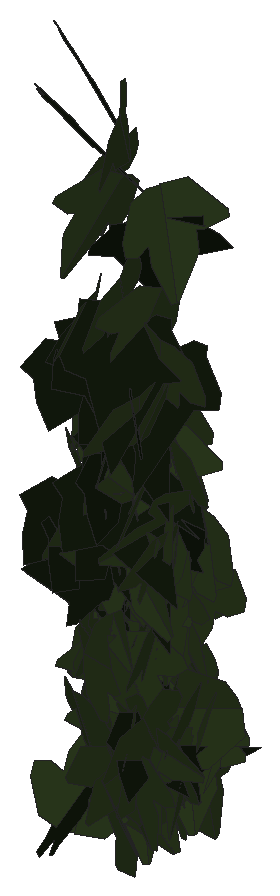
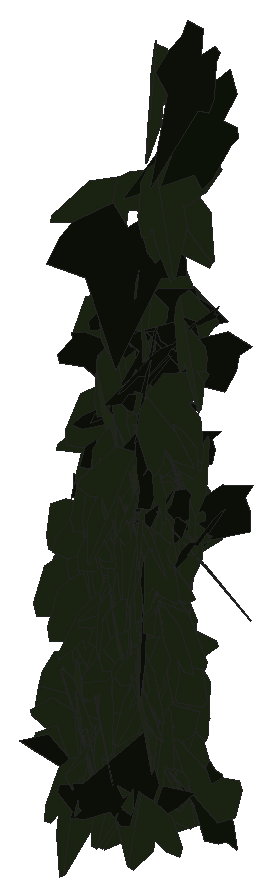
# SketchUp Ruby script. Lengths in inches.
U = 1.inch
M = Sketchup.active_model
def pt(a) = Geom::Point3d.new(a.map { |v| v * U })
def face(e, loops, mat)
  f = e.add_face(loops[0].map { |a| pt(a) })
  loops[1..].each { |l| e.add_face(l.map { |a| pt(a) }).erase! }
  f.material = f.back_material = mat if mat
  f
end
# faces: each face lists its corners as indices into pts; further lists are holes
def faces(e, pts, list, mat = nil) = list.each { |f| face(e, (f[0].is_a?(Array) ? f : [f]).map { |l| l.map { |i| pts[i] } }, mat) }
# xy, xz, yz: faces in a plane at the given z, y or x. An outline is a flat list of corners, or four numbers for a rectangle; further outlines are holes
def ring(l) = l.size == 4 ? [[l[0], l[1]], [l[2], l[1]], [l[2], l[3]], [l[0], l[3]]] : l.each_slice(2).to_a
def flat(e, list, mat, &to3) = list.each { |f| face(e, (f[0].is_a?(Array) ? f : [f]).map { |l| ring(l).map { |u, v| to3.(u, v) } }, mat) }
def xy(e, z, list, mat = nil) = flat(e, list, mat) { |x, y| [x, y, z] }
def xz(e, y, list, mat = nil) = flat(e, list, mat) { |x, z| [x, y, z] }
def yz(e, x, list, mat = nil) = flat(e, list, mat) { |y, z| [x, y, z] }
def lines(e, pts, list) = list.each { |a, b| e.add_line(pt(pts[a]), pt(pts[b])) }
# prism: a flat outline (further loops are holes) pulled along v
def prism(e, loops, v, mat = nil)
  f = face(e, loops, mat); d = Geom::Vector3d.new(v.map { |x| x * U })
  f.pushpull(f.normal.samedirection?(d) ? d.length : -d.length)
end
def box(e, o, s, mat = nil) = prism(e, [[o, [o[0] + s[0], o[1], o[2]], [o[0] + s[0], o[1] + s[1], o[2]], [o[0], o[1] + s[1], o[2]]]], [0, 0, s[2]], mat)
def at(x, y, z, deg = 0) = Geom::Transformation.translation(pt([x, y, z])) * Geom::Transformation.rotation(ORIGIN, Z_AXIS, deg.degrees)
def axes(o, x, y, z) = Geom::Transformation.new([*x, 0, *y, 0, *z, 0, *pt(o).to_a, 1])
def part(name) = M.definitions.add(name)
# library, detail: a bought-in or finely detailed component or shape, given as its bounding box
def library(name, o, s) = part(name).tap { |d| box(d.entities, o, s) }
def detail(e, o, s) = box(e.add_group.entities, o, s)
def put(e, d, t, mat = nil) = e.add_instance(d, t).tap { |i| i.material = mat if mat }
def group(e, t, mat = nil) = e.add_group.tap { |g| g.transformation = t; g.material = mat if mat }.entities
root = M.entities
M.materials.add("efeu1").color = [18, 25, 13]
M.materials.add("efeu2").color = [43, 57, 29]
c1 = part("ivyleaf_10")
p = [[0,0.5,-0.03],[-0.0625,2.02,-0.43],[-0.19,2.01,-0.46],[-0.54,1.05,-0.29],[-0.52,0.625,-0.18],[-0.83,0.76,-0.28],
  [-1.16,0.64,-0.33],[-1.15,0.33,-0.24],[-0.77,-0.39,0.02],[-0.3,-0.51,0.16],[0.04,-0.48,0.23],[-0.02,2.01,-0.4375],
  [-0.06,2.01,-0.43],[0.04,-0.49,0.23],[0.67,-0.49,0.14],[1.38,0.36,-0.2],[1.375,0.51,-0.24],[0.81,0.65,-0.19],
  [0.62,0.59,-0.15],[0.6,1.09,-0.28],[0.5,1.23,-0.31]]
faces(c1.entities,p,[[0,1,2,3,4,5,6,7,8,9,10],[11,12,0,13,14,15,16,17,18,19,20]],"efeu2")
c2 = part("ivyleaf_9")
p = [[1.54,2.16,1.25],[1.36,2.04,1.19],[-0.21,0.99,0.68],[-0.71,1.11,0.82],[-0.85,0.86,0.67],[-0.8,0.17,0.21],
  [-0.9,-0.01,0.1],[-0.67,-0.16,-0.02],[-0.08,-0.08,-0.05],[-0.03,-0.6,-0.4],[0.65,-0.88,-0.66],[0.83,-0.6,-0.49],
  [1.29,-0.42,-0.43],[1.8125,-0.07,-0.26],[1.21,0.44,0.15]]
faces(c2.entities,p,[[0,1,2,3,4,5,6,7,8,9,10,11,12,13,14]],"efeu1")
put(root,c1,axes([21.54,225.2,216.51],[0.41604,-0.27169,0.05558],[0.08058,0.02255,-0.49295],[0.26536,0.41913,0.06255]))
put(root,c1,axes([21.65,225.15,219.01],[0.01266,-0.40962,0.28645],[0.04495,-0.28445,-0.40874],[0.49781,0.0361,0.02962]))
put(root,c1,axes([21.73,225.11,215.11],[-0.42278,0.2511,0.09058],[-0.10121,0.00622,-0.48961],[-0.24701,-0.43233,0.04557]))
put(root,c1,axes([21.71,225.37,215.82],[0.1972,-0.44181,-0.12615],[-0.03153,0.12394,-0.48337],[0.45839,0.1986,0.02102]))
put(root,c1,axes([21.59,225.14,215.95],[-0.16549,-0.37731,-0.28328],[0.18997,0.22151,-0.40601],[0.43188,-0.24201,0.07005]))
put(root,c1,axes([21.7,224.63,219.89],[0.14778,-0.47571,-0.04311],[0.00221,0.0458,-0.49789],[0.47766,0.14696,0.01564]))
put(root,c1,axes([21.59,224.64,213.92],[0.38502,0.29053,-0.13174],[0.10689,0.07705,0.48233],[0.30056,-0.39957,-0.00277]))
put(root,c2,axes([21.44,224.42,222.3125],[0.47565,-0.15225,-0.02409],[-0.00548,0.06139,-0.49619],[0.15404,0.47228,0.05674]))
put(root,c1,axes([21.7,225.26,216.42],[-0.39747,-0.26793,-0.14223],[0.10687,0.09572,-0.47898],[0.28389,-0.41116,-0.01882]))
put(root,c1,axes([21.74,224.64,217.54],[-0.04796,-0.48317,-0.11937],[0.03109,0.11678,-0.48518],[0.49672,-0.05396,0.01884]))
put(root,c2,axes([21.59,224.6,217.65],[-0.01697,-0.37042,-0.33541],[-0.00806,0.33576,-0.3704],[0.49965,-0.00717,-0.01737]))
put(root,c2,axes([21.69,224.17,213.86],[-0.20042,0.45805,-0.0044],[-0.00475,0.00272,0.49997],[0.45805,0.20045,0.00326]))
put(root,c1,axes([22.02,224.84,217.42],[0.04947,0.04496,-0.49551],[-0.32133,0.38307,0.00268],[0.37987,0.31818,0.06679]))
put(root,c2,axes([21.71,224.43,222.99],[0.40824,-0.03682,-0.28633],[-0.28129,0.06078,-0.40888],[0.06492,0.49492,0.02891]))
put(root,c1,axes([21.82,225.16,214.95],[-0.14194,-0.42822,0.21559],[-0.00134,-0.22449,-0.44677],[0.47943,-0.12741,0.06258]))
put(root,c2,axes([21.57,224.68,217.2],[0.22108,-0.41378,-0.17295],[-0.08343,0.15151,-0.46913],[0.44064,0.23629,-0.00205]))
put(root,c1,axes([21.81,224.63,216.55],[0.04249,0.01142,-0.49806],[-0.00091,0.49987,0.01138],[0.49819,-0.00006,0.0425]))
put(root,c2,axes([21.97,224.96,216.85],[0.06294,-0.03259,-0.49495],[-0.45396,0.19727,-0.07072],[0.19989,0.45828,-0.00476]))
put(root,c1,axes([21.75,224.89,215.46],[-0.19102,0.45911,0.0522],[-0.01529,0.05018,-0.49724],[-0.46182,-0.19156,-0.00513]))
put(root,c1,axes([21.78,225.29,217.32],[-0.49192,0.07312,-0.05167],[0.04949,-0.01842,-0.4972],[-0.07462,-0.49428,0.01088]))
put(root,c1,axes([21.84,224.9,221.59],[0.02564,-0.49813,-0.03474],[-0.00713,0.03442,-0.49876],[0.49929,0.02607,-0.00533]))
put(root,c1,axes([21.71,225.31,215.92],[0.35958,-0.34514,0.03978],[0.09029,0.03755,-0.49035],[0.33549,0.35982,0.08933]))
put(root,c1,axes([21.81,224.4375,215.25],[-0.44392,0.23002,-0.00536],[0.00529,-0.00145,-0.49997],[-0.23002,-0.44395,-0.00115]))
put(root,c2,axes([22.15,224.38,217.12],[-0.34255,0.29401,0.21497],[-0.17815,0.12215,-0.45093],[-0.31768,-0.38553,0.02107]))
put(root,c1,axes([21.74,225.46,215.76],[0.38872,-0.28553,0.13181],[0.10715,-0.07677,-0.48231],[0.29567,0.40321,0.00151]))
put(root,c1,axes([21.55,224.7,217.75],[-0.13534,-0.00274,0.48133],[0.44109,-0.20086,0.12288],[0.19268,0.45787,0.05679]))
put(root,c1,axes([21.92,224.92,215.84],[-0.17482,-0.44912,0.13316],[0.01365,-0.14695,-0.47772],[0.46824,-0.1634,0.06364]))
put(root,c1,axes([21.88,225.1875,216.64],[0.14766,-0.46817,-0.09494],[0.01371,0.10348,-0.48898],[0.4775,0.1418,0.0434]))
put(root,c1,axes([21.93,224.7,221.32],[-0.03902,-0.42987,0.25238],[-0.0208,-0.25152,-0.43163],[0.49804,-0.04418,0.00175]))
put(root,c2,axes([22.04,225.5,214.16],[-0.41951,-0.23548,0.13624],[0.13386,0.03932,0.48014],[-0.23684,0.43932,0.03005]))
put(root,c1,axes([21.84,225.3,216.17],[0.12222,0.48453,-0.01723],[-0.05019,-0.00503,-0.49745],[-0.48223,0.12332,0.04741]))
put(root,c1,axes([22.16,224.96,218.28],[-0.42118,0.09296,0.25292],[-0.26479,-0.05576,-0.42045],[-0.04996,-0.48811,0.0962]))
put(root,c1,axes([21.82,224.63,215.86],[-0.24361,0.28524,0.33059],[0.22257,-0.24457,0.37503],[0.37566,0.32988,-0.00782]))
put(root,c1,axes([21.99,224.77,217.17],[-0.19886,-0.45215,0.07755],[0.00778,-0.08783,-0.49216],[0.45869,-0.19454,0.04196]))
put(root,c1,axes([21.92,225.14,217.04],[0.14819,-0.44913,-0.16223],[0.05568,0.18496,-0.46118],[0.47428,0.11862,0.10483]))
put(root,c1,axes([22,224.88,216.875],[0.446,-0.17424,-0.14396],[-0.13368,0.05342,-0.47883],[0.18224,0.4656,0.00107]))
put(root,c1,axes([21.98,224.76,216.26],[-0.02511,-0.43788,-0.24007],[0.01663,0.23951,-0.43859],[0.49909,-0.03002,0.00253]))
put(root,c1,axes([21.91,225.125,217.48],[0.3805,-0.32173,0.04135],[0.04906,-0.00593,-0.49755],[0.32065,0.38269,0.02706]))
put(root,c1,axes([22.02,225.25,216.35],[-0.02831,-0.49885,-0.01868],[0.0001,0.0187,-0.49965],[0.4992,-0.02829,-0.00096]))
put(root,c2,axes([21.74,224.44,219.53],[0.05321,-0.24019,-0.43529],[0.09638,0.43445,-0.22795],[0.48773,-0.05965,0.09253]))
put(root,c1,axes([21.78,225.31,214.19],[0.4614,-0.02549,0.19095],[0.19141,0.00459,-0.46189],[0.0218,0.49933,0.01399]))
put(root,c1,axes([22.0625,224.99,217.7],[-0.31177,-0.39089,-0.00275],[0.00995,-0.00442,-0.49988],[0.39077,-0.31175,0.01053]))
put(root,c2,axes([21.9375,224.84,217.9375],[-0.00466,0.26312,0.42514],[-0.12666,-0.41191,0.25355],[0.48367,-0.10533,0.07049]))
put(root,c1,axes([22.03,225.13,216.61],[0.48608,0.07074,-0.09341],[-0.09849,0.03068,-0.48924],[-0.06349,0.49402,0.04376]))
put(root,c1,axes([22.08,225.24,216.47],[-0.02487,-0.49921,0.0131],[0.00115,-0.01317,-0.49983],[0.49938,-0.02483,0.0018]))
put(root,c1,axes([21.92,225.17,217.76],[-0.14664,0.1767,-0.44416],[0.10151,-0.44248,-0.20954],[-0.46711,-0.15163,0.0939]))
put(root,c1,axes([22.09,224.51,218.72],[0.28079,-0.39602,-0.11967],[-0.04583,0.11397,-0.48468],[0.41117,0.28315,0.0277]))
put(root,c1,axes([22.15,225.05,217.32],[-0.38317,-0.31931,0.0349],[-0.02507,-0.02443,-0.49877],[0.32023,-0.38398,0.00271]))
put(root,c2,axes([21.875,224.65,219.53],[0.10076,-0.4835,-0.07796],[0.00208,0.08001,-0.49355],[0.48974,0.09913,0.01813]))
put(root,c1,axes([22.1,225.25,218.15],[-0.03135,0.41855,0.27173],[-0.09556,0.26219,-0.41488],[-0.48978,-0.07795,0.06356]))
put(root,c1,axes([22.18,224.21,216.06],[-0.1022,0.29197,0.39282],[-0.17579,0.35262,-0.30782],[-0.45679,-0.20102,0.03058]))
put(root,c1,axes([22.05,224.96,217.98],[-0.23027,0.44236,-0.03594],[0.01753,-0.03139,-0.49871],[-0.44347,-0.23093,-0.00105]))
put(root,c1,axes([22.09,224.8125,217.33],[0.45247,0.18716,-0.1012],[-0.09055,-0.04582,-0.48959],[-0.19254,0.46138,-0.00757]))
put(root,c1,axes([22.39,224.37,213.96],[-0.07021,0.15328,-0.47072],[-0.31966,0.34899,0.16132],[0.378,0.32359,0.04899]))
put(root,c1,axes([21.83,224.87,218.62],[0.39549,0.03178,0.30426],[0.30399,0.01492,-0.39669],[-0.03429,0.49877,-0.00752]))
put(root,c1,axes([22.17,225.25,215.83],[-0.08288,-0.47592,-0.12897],[0.01114,0.12894,-0.48296],[0.49296,-0.08293,-0.01077]))
put(root,c1,axes([21.78,224.69,216.61],[0.23796,-0.06985,0.43416],[0.42215,-0.10194,-0.24778],[0.12313,0.48449,0.01046]))
put(root,c1,axes([22.03,224.88,214.32],[-0.42866,-0.14827,-0.21039],[0.20514,0.05004,-0.45323],[0.15545,-0.47488,0.01793]))
put(root,c1,axes([22.22,225.06,218.35],[-0.1226,-0.47129,0.11339],[-0.01963,-0.11204,-0.48689],[0.48434,-0.12384,0.00897]))
put(root,c1,axes([22.19,224.625,215.23],[0.34469,-0.34487,-0.1107],[-0.07468,0.08186,-0.48757],[0.35442,0.35265,0.00492]))
put(root,c1,axes([22.17,225.2,216.4375],[0.21506,-0.44952,-0.04094],[-0.01367,0.03884,-0.4983],[0.45118,0.21545,0.00441]))
put(root,c1,axes([22.23,225.13,217.92],[-0.16375,-0.46516,0.08251],[-0.01503,-0.08215,-0.49298],[0.47219,-0.16393,0.01292]))
put(root,c1,axes([22.34,225.17,214.9],[0.08674,0.21292,0.44401],[-0.17962,-0.4061,0.22983],[0.45849,-0.19938,0.00604]))
put(root,c1,axes([22.09,224.71,216.41],[0.04888,-0.04987,0.4951],[0.00699,0.4975,0.04942],[-0.49756,0.00209,0.04933]))
put(root,c1,axes([22.2,224.52,220.34],[0.04565,-0.44879,-0.21565],[0.01783,0.21789,-0.44967],[0.49759,0.03337,0.03589]))
put(root,c2,axes([22.33,224.7,218.67],[0.08352,-0.27264,0.41072],[-0.03646,0.41202,0.28091],[-0.49163,-0.07687,0.04894]))
put(root,c1,axes([22.23,225.2,214.52],[-0.44388,0.23015,-0.00025],[0.00038,0.00018,-0.5],[-0.23015,-0.44388,-0.00033]))
put(root,c2,axes([22.3,224.92,220.88],[0.24312,0.40368,-0.16714],[-0.10135,-0.13395,-0.47094],[-0.425,0.26287,0.01669]))
put(root,c2,axes([22.18,224.46,218.35],[0.17597,-0.25481,-0.39256],[-0.20248,0.33666,-0.30929],[0.42194,0.26783,0.01529]))
put(root,c2,axes([22.27,224.96,217.1875],[0.40763,-0.11085,0.26749],[-0.24336,0.11911,0.42022],[-0.15688,-0.47278,0.04315]))
put(root,c1,axes([22.23,224.48,214.77],[-0.45168,-0.16143,-0.14117],[0.12932,0.05754,-0.47955],[0.17107,-0.46971,-0.01023]))
put(root,c2,axes([22.09,224.79,217.45],[0.07264,-0.45036,-0.20469],[-0.01292,0.20509,-0.45582],[0.49453,0.07151,0.01816]))
put(root,c1,axes([22.34,224.73,217.97],[0.20427,-0.43715,-0.13107],[-0.05576,0.11861,-0.48252],[0.45295,0.21174,-0.00029]))
put(root,c1,axes([22.23,224.58,216.02],[-0.44824,-0.17574,-0.13488],[0.14252,0.0043,-0.47924],[0.1696,-0.46808,0.04624]))
put(root,c1,axes([22.28,224.59,214.6875],[-0.47691,0.1415,-0.05038],[0.0464,-0.0207,-0.49741],[-0.14285,-0.47911,0.00661]))
put(root,c1,axes([22.33,225.12,218.08],[0.13572,-0.48032,-0.02952],[0.0052,0.03214,-0.49894],[0.4812,0.13513,0.01372]))
put(root,c1,axes([22.27,224.97,217.53],[0.34796,-0.35733,0.0352],[0.04745,-0.00283,-0.49774],[0.35591,0.34972,0.03194]))
put(root,c1,axes([22.31,225.375,215.39],[0.25739,-0.42859,-0.00793],[0.0242,0.02376,-0.49885],[0.42798,0.25641,0.03297]))
put(root,c1,axes([22.37,225.15,217.64],[0.3631,-0.29313,-0.17953],[-0.08038,0.1815,-0.45891],[0.33421,0.36212,0.08468]))
put(root,c2,axes([22.14,224.75,219.07],[0.09432,-0.45829,-0.17627],[-0.02182,0.1754,-0.46772],[0.49054,0.09592,0.01308]))
put(root,c1,axes([22.42,224.92,218.7],[-0.39362,-0.30454,0.04813],[-0.04489,-0.02061,-0.49755],[0.30504,-0.39602,-0.01112]))
put(root,c1,axes([22.4,225,217.81],[-0.25708,-0.41961,0.08852],[-0.01291,-0.09559,-0.49061],[0.42865,-0.25454,0.03831]))
put(root,c1,axes([22.02,224.92,217.1],[-0.10794,0.05715,-0.48485],[0.36446,-0.32096,-0.11897],[-0.32483,-0.37911,0.02763]))
put(root,c1,axes([22.43,225.28,214.62],[0.0544,0.12958,-0.47984],[-0.06004,0.48089,0.12305],[0.49339,0.04423,0.06788]))
put(root,c1,axes([22.3,224.54,214.67],[-0.15553,-0.36467,-0.30468],[0.13203,0.2748,-0.3963],[0.45649,-0.20373,0.01082]))
put(root,c1,axes([22.35,225.13,217.28],[-0.45894,-0.19098,-0.05386],[0.08106,-0.05659,-0.49013],[0.18111,-0.45861,0.0829]))
put(root,c1,axes([22.4,224.9,219.22],[-0.01518,-0.49972,0.00699],[0.00176,-0.00705,-0.49995],[0.49977,-0.01515,0.00198]))
put(root,c1,axes([22.4,224.81,220.08],[-0.05412,-0.45777,0.19369],[0.01357,-0.19612,-0.45973],[0.49688,-0.04451,0.03365]))
put(root,c1,axes([22.37,225.23,216.98],[-0.49557,-0.02498,-0.06154],[0.06478,-0.07955,-0.48936],[0.01466,-0.493,0.08208]))
put(root,c2,axes([22.3125,224.57,219.83],[-0.27336,-0.38628,-0.16144],[0.08008,0.14101,-0.47297],[0.41093,-0.28444,-0.01522]))
put(root,c1,axes([22.4375,224.21,222.55],[0.14975,-0.3708,-0.30014],[-0.04023,0.30364,-0.3952],[0.47535,0.14251,0.06111]))
put(root,c1,axes([22.35,225.09,217.07],[0.47343,-0.16081,-0.00274],[-0.00253,0.00109,-0.49999],[0.16081,0.47343,0.00022]))
put(root,c1,axes([22.3125,224.4,218.13],[-0.1686,-0.33902,-0.32656],[0.1841,0.27175,-0.37717],[0.43322,-0.24742,0.0332]))
put(root,c1,axes([22.26,225.22,216.46],[-0.41275,0.16853,-0.22636],[0.20309,-0.1011,-0.44557],[-0.19595,-0.45976,0.015]))
put(root,c2,axes([22.07,224.75,214.38],[0.19351,0.03418,0.45977],[0.43658,0.14667,-0.19465],[-0.14817,0.47678,0.02692]))
put(root,c1,axes([22.35,225.34,216.51],[0.01763,0.45253,-0.2119],[-0.00697,-0.21179,-0.45287],[-0.49964,0.01892,-0.00116]))
put(root,c1,axes([22.44,225.04,214.77],[0.06588,-0.30342,-0.39192],[0.02119,0.39672,-0.30358],[0.49519,0.02339,0.06513]))
put(root,c2,axes([22.1875,224.43,218.08],[0.04499,-0.4087,-0.28449],[0.09316,0.28752,-0.39831],[0.48918,-0.01716,0.10202]))
put(root,c1,axes([22.47,224.78,216.3125],[0.14112,-0.44068,-0.18944],[-0.03326,0.188,-0.46211],[0.47852,0.14302,0.02375]))
put(root,c1,axes([22.49,225.25,216.51],[-0.26225,-0.4235,0.04325],[0.01454,-0.05968,-0.49621],[0.42546,-0.259,0.04362]))
put(root,c2,axes([22.23,224.72,218.61],[0.01218,-0.32777,-0.37738],[0.07175,0.37473,-0.32315],[0.49467,-0.04629,0.05616]))
put(root,c1,axes([22.45,225.23,217.09],[0.4865,-0.07372,-0.08879],[-0.08253,0.04664,-0.49093],[0.08067,0.49233,0.03321]))
put(root,c2,axes([22.39,224.64,215.28],[0.19725,-0.23514,-0.39472],[-0.23324,0.31884,-0.3065],[0.39585,0.30503,0.01609]))
put(root,c1,axes([22.49,225.01,219.07],[0.19131,-0.46082,-0.03229],[-0.01055,0.03058,-0.49895],[0.46183,0.19159,0.00197]))
put(root,c1,axes([22.4375,224.8,217.66],[0.44435,-0.22917,0.00562],[0.00504,-0.0025,-0.49997],[0.22919,0.44438,0.00009]))
put(root,c1,axes([22.6,225.47,215.38],[0.30843,-0.34603,-0.18744],[-0.13353,0.13201,-0.46341],[0.37019,0.33592,-0.01098]))
put(root,c1,axes([22.64,224.71,219.63],[-0.47898,0.06033,0.13014],[-0.13367,-0.02321,-0.48124],[-0.05202,-0.4958,0.03836]))
put(root,c1,axes([22.56,224.38,219.11],[-0.10281,-0.47737,-0.10747],[0.01084,0.10757,-0.48817],[0.4892,-0.10271,-0.01177]))
put(root,c1,axes([22.67,225.31,217.34],[-0.45904,0.14946,0.13016],[-0.16665,-0.11336,-0.45758],[-0.10727,-0.46348,0.15389]))
put(root,c2,axes([22.49,224.94,219.45],[-0.33537,-0.33511,-0.15882],[0.11218,0.11243,-0.4741],[0.35347,-0.35364,-0.00022]))
put(root,c1,axes([22.87,225.29,215.24],[0.06262,0.07669,-0.4901],[-0.49094,-0.06121,-0.0723],[-0.07108,0.49028,0.06763]))
put(root,c1,axes([22.52,225.49,214.3125],[-0.03712,-0.47685,-0.14573],[0.06895,0.13982,-0.47507],[0.49383,-0.05537,0.05538]))
put(root,c1,axes([22.49,224.79,214.69],[-0.16759,-0.34225,-0.32369],[0.13619,0.29369,-0.38105],[0.45096,-0.21589,-0.00521]))
put(root,c1,axes([22.625,225.23,215.36],[0.15345,-0.44362,-0.1722],[-0.05439,0.16339,-0.46941],[0.47275,0.1628,0.00189]))
put(root,c1,axes([22.47,224.79,218.4],[0.29064,0.40685,-0.00023],[-0.00015,-0.00017,-0.5],[-0.40685,0.29064,0.00002]))
put(root,c1,axes([22.39,225.34,214.72],[0.45576,0.16555,0.12198],[0.11616,0.03746,-0.48487],[-0.16968,0.47031,-0.00432]))
put(root,c1,axes([22.61,224.45,215.33],[-0.07256,-0.42038,-0.2608],[0.03532,0.25851,-0.42652],[0.49344,-0.08032,-0.00782]))
put(root,c1,axes([22.23,224.54,217.1875],[0.28955,-0.01231,0.40744],[0.40757,0.01704,-0.28913],[-0.00677,0.49956,0.0199]))
put(root,c1,axes([22.63,224.94,218.36],[-0.42411,0.25999,0.05036],[-0.05829,0.0011,-0.49659],[-0.25832,-0.42709,0.02937]))
put(root,c1,axes([22.45,225.33,214.7],[0.07056,-0.3703,0.32848],[0.22713,-0.27058,-0.35383],[0.43981,0.19915,0.13003]))
put(root,c1,axes([22.67,225.21,216.71],[-0.34134,-0.35606,0.08187],[-0.00315,-0.10917,-0.48793],[0.36534,-0.33362,0.07228]))
put(root,c1,axes([22.47,225.51,215.02],[0.4932,0.03474,0.07445],[0.07519,-0.00826,-0.49425],[-0.03311,0.49872,-0.01337]))
put(root,c1,axes([22.75,224.91,217.6],[-0.02654,0.12428,-0.48358],[-0.27125,-0.41016,-0.09052],[-0.41919,0.25753,0.08919]))
put(root,c1,axes([22.67,224.7,217.39],[0.04519,-0.49779,-0.01291],[-0.00316,0.01267,-0.49983],[0.49794,0.04526,-0.002]))
put(root,c1,axes([22.54,224.86,221.27],[0.18463,0.4639,0.02668],[0.00959,0.0249,-0.49929],[-0.46457,0.18488,0.00029]))
put(root,c1,axes([22.27,224.71,214.95],[-0.01025,-0.07065,0.49488],[0.49868,0.03306,0.01505],[-0.03485,0.49388,0.06978]))
